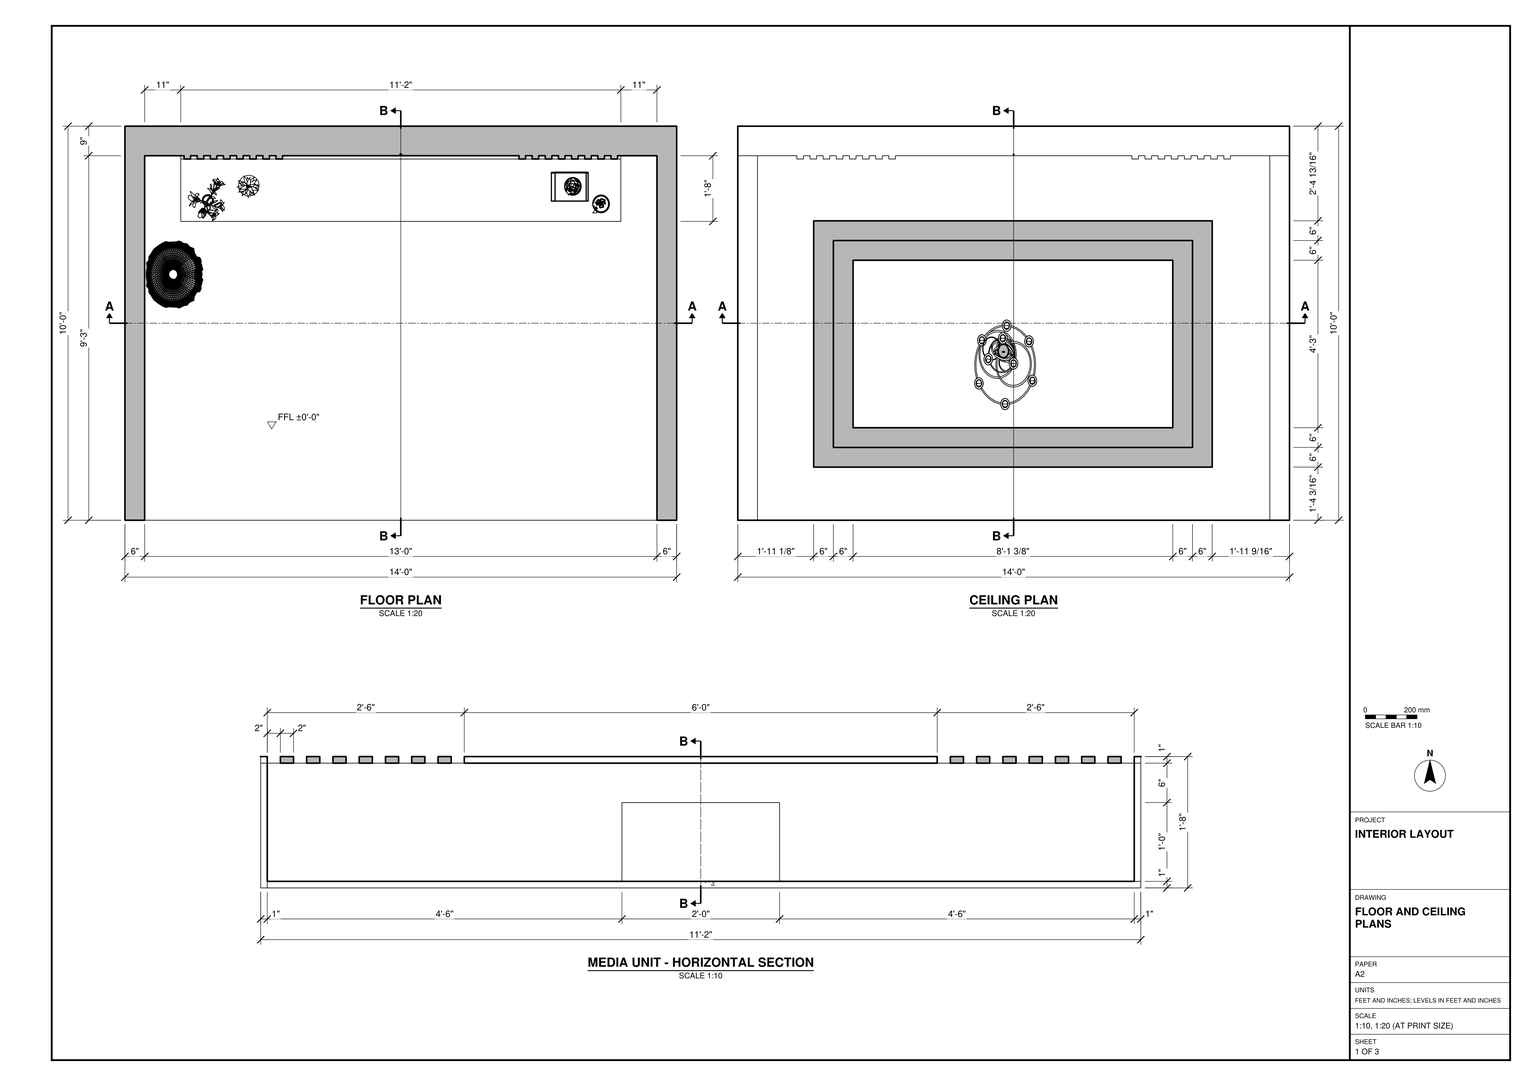
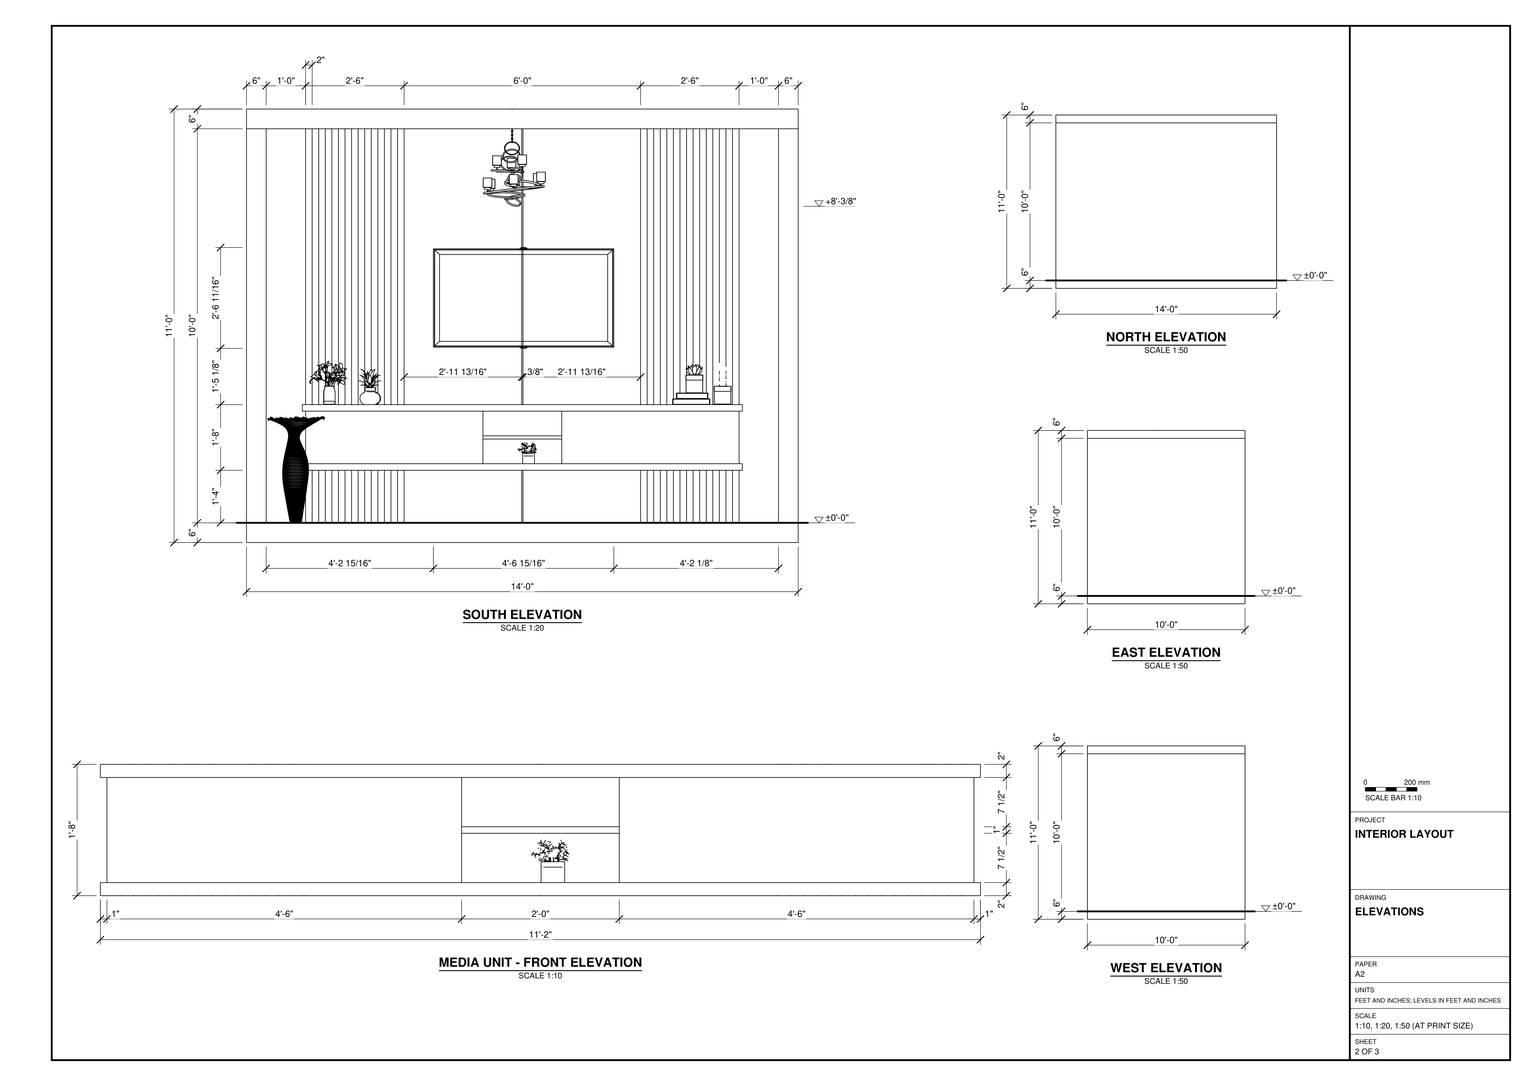
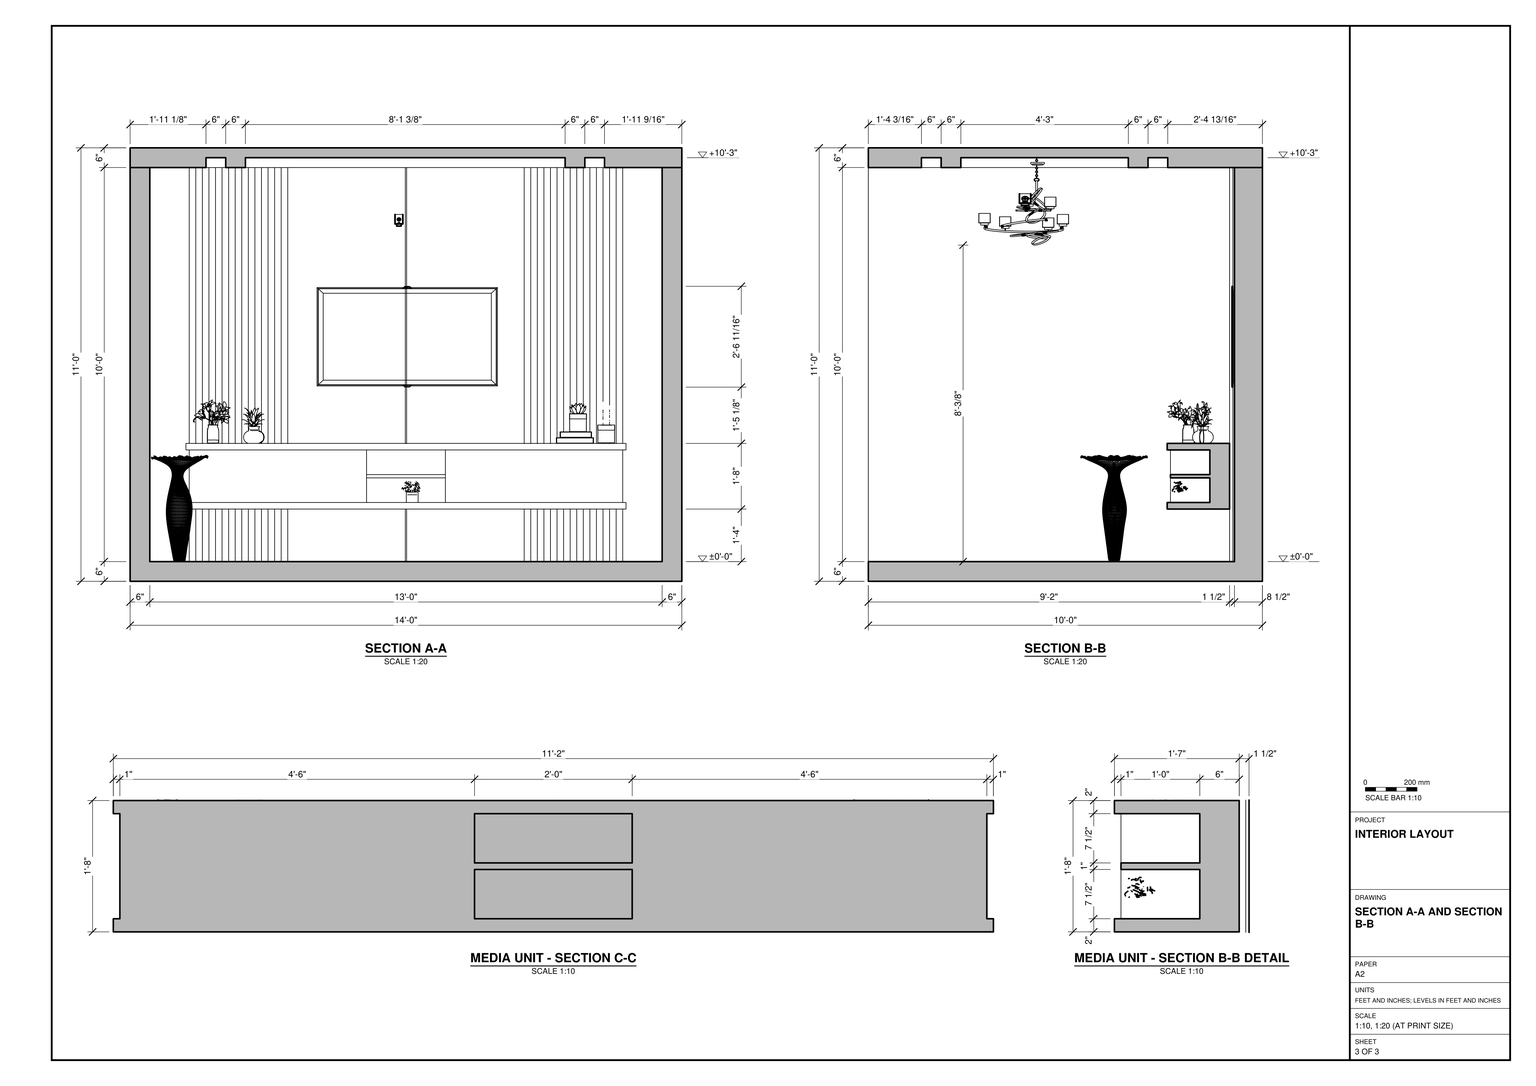
Build the room in SketchUp from task_files/diagram_01.pdf. Work in feet and inches. The room is 14'-0" wide, 10'-0" deep and 11'-0" high overall. Use the finished floor at ±0'-0" as the datum. Model the floor slab, the two 6" side walls and the rear wall assembly shown as 9" thick in plan. Leave the front open as drawn. Shape the underside of the ceiling slab to form the rectangular recess and its stepped border, following the ceiling plan and both sections.

On the rear wall, place the screen on the broad central panel between fields of vertical slats. Continue the panel and slat pattern below the floating media unit. Centre the 11'-2" unit across the wall with its underside 1'-4" above the finished floor. Use the enlarged joinery details to set out the projecting top and bottom boards, the broad side bays and the shelf dividing the open middle bay. Place the hanging light in the ceiling recess, the floor vase to the left of the unit and the smaller display items as shown in elevation. Decor and loose items may be any suitable library components.

Keep the walls, floor slab and ceiling slab as separate groups or components, and do the same for each furniture or joinery piece. Use components for repeated parts such as the slats. Save one SketchUp model as output_files/media_room_with_floating_joinery_and_a_recessed_ceiling.skp.

# SketchUp Ruby script. Lengths in inches.
U = 1.inch
M = Sketchup.active_model
def pt(a) = Geom::Point3d.new(a.map { |v| v * U })
def face(e, loops, mat)
  f = e.add_face(loops[0].map { |a| pt(a) })
  loops[1..].each { |l| e.add_face(l.map { |a| pt(a) }).erase! }
  f.material = f.back_material = mat if mat
  f
end
# faces: each face lists its corners as indices into pts; further lists are holes
def faces(e, pts, list, mat = nil) = list.each { |f| face(e, (f[0].is_a?(Array) ? f : [f]).map { |l| l.map { |i| pts[i] } }, mat) }
# xy, xz, yz: faces in a plane at the given z, y or x. An outline is a flat list of corners, or four numbers for a rectangle; further outlines are holes
def ring(l) = l.size == 4 ? [[l[0], l[1]], [l[2], l[1]], [l[2], l[3]], [l[0], l[3]]] : l.each_slice(2).to_a
def flat(e, list, mat, &to3) = list.each { |f| face(e, (f[0].is_a?(Array) ? f : [f]).map { |l| ring(l).map { |u, v| to3.(u, v) } }, mat) }
def xy(e, z, list, mat = nil) = flat(e, list, mat) { |x, y| [x, y, z] }
def xz(e, y, list, mat = nil) = flat(e, list, mat) { |x, z| [x, y, z] }
def yz(e, x, list, mat = nil) = flat(e, list, mat) { |y, z| [x, y, z] }
def lines(e, pts, list) = list.each { |a, b| e.add_line(pt(pts[a]), pt(pts[b])) }
# prism: a flat outline (further loops are holes) pulled along v
def prism(e, loops, v, mat = nil)
  f = face(e, loops, mat); d = Geom::Vector3d.new(v.map { |x| x * U })
  f.pushpull(f.normal.samedirection?(d) ? d.length : -d.length)
end
def box(e, o, s, mat = nil) = prism(e, [[o, [o[0] + s[0], o[1], o[2]], [o[0] + s[0], o[1] + s[1], o[2]], [o[0], o[1] + s[1], o[2]]]], [0, 0, s[2]], mat)
def at(x, y, z, deg = 0) = Geom::Transformation.translation(pt([x, y, z])) * Geom::Transformation.rotation(ORIGIN, Z_AXIS, deg.degrees)
def axes(o, x, y, z) = Geom::Transformation.new([*x, 0, *y, 0, *z, 0, *pt(o).to_a, 1])
def part(name) = M.definitions.add(name)
# library, detail: a bought-in or finely detailed component or shape, given as its bounding box
def library(name, o, s) = part(name).tap { |d| box(d.entities, o, s) }
def detail(e, o, s) = box(e.add_group.entities, o, s)
def put(e, d, t, mat = nil) = e.add_instance(d, t).tap { |i| i.material = mat if mat }
def group(e, t, mat = nil) = e.add_group.tap { |g| g.transformation = t; g.material = mat if mat }.entities
root = M.entities
M.materials.add("[0030_OldLace]").color = [253, 245, 230]
M.materials.add("[Carrera Marble]").color = [207, 207, 207]
M.materials.add("[Wood Bamboo]").color = [177, 105, 43]
c1 = library("Flat screen television",[0,1.41,1.14],[35.92,0.28,20.21])
c2 = library("Mint+Plant",[-0.84,-3.51,-0.07],[7.9,7.03,9.76])
c3 = library("suculentas com livro",[0,-0.27,0],[14.84,10.07,7.14])
c4 = library("lọ hoa",[2.76,5.43,0],[11.3,13.25,13.27])
c5 = library("MORNING+GLORY_AQUA",[22.86,12.49,0.11],[41.56,45.92,85.24])
c6 = library("Group_432",[-8.27,-1.37,0],[9.69,9.67,11.03])
c7 = library("Dalen+Chandelier",[-1.89,-23.41,-0.83],[35.87,36,58.86])
xy(root,126,[[[0,0,168,120],[23.11,16.17,144.46,91.17]],[[29.11,22.17,138.46,85.17],[35.11,28.17,132.46,79.17]]],"[0030_OldLace]")
xy(root,129,[[[23.11,16.17,144.46,91.17],[29.11,22.17,138.46,85.17]],[35.11,28.17,132.46,79.17]],"[0030_OldLace]")
xy(root,132,[[0,0,168,120]],"[0030_OldLace]")
xz(root,0,[[0,126,168,132]],"[0030_OldLace]")
xz(root,16.17,[[23.11,126,144.46,129]],"[0030_OldLace]")
xz(root,22.17,[[29.11,126,138.46,129]],"[0030_OldLace]")
xz(root,28.17,[[35.11,126,132.46,129]],"[0030_OldLace]")
xz(root,79.17,[[35.11,126,132.46,129]],"[0030_OldLace]")
xz(root,85.17,[[29.11,126,138.46,129]],"[0030_OldLace]")
xz(root,91.17,[[23.11,126,144.46,129]],"[0030_OldLace]")
xz(root,120,[[0,126,168,132]],"[0030_OldLace]")
yz(root,0,[[0,126,120,132]],"[0030_OldLace]")
yz(root,23.11,[[16.17,126,91.17,129]],"[0030_OldLace]")
yz(root,29.11,[[22.17,126,85.17,129]],"[0030_OldLace]")
yz(root,35.11,[[28.17,126,79.17,129]],"[0030_OldLace]")
yz(root,132.46,[[28.17,126,79.17,129]],"[0030_OldLace]")
yz(root,138.46,[[22.17,126,85.17,129]],"[0030_OldLace]")
yz(root,144.46,[[16.17,126,91.17,129]],"[0030_OldLace]")
yz(root,168,[[0,126,120,132]],"[0030_OldLace]")
put(root,c1,axes([56.91,109.3125,57.4],[1.52975,0,0],[0,1,0],[0,0,1.5196]))
put(root,c2,axes([83.13,94.06,24.05],[0.78,0,0],[0,0.87,0],[0,0,0.69]))
put(root,c3,axes([129.76,93.57,42],[1.2,0,0],[0,1.27693,0],[0,0,2]))
put(root,c4,at(16.47,85.57,42))
put(root,c5,axes([-3.04,59.05,5.96],[0.416,0,0],[0,0.445,0],[0,0,0.38]))
put(root,c6,at(40.92,98.19,42))
put(root,c7,axes([71.87,51.53,102.26],[0.59559,0,0],[0,0.77552,0],[0,0,0.51254]))
g1 = group(root,at(0,0,0),"[0030_OldLace]")
xy(g1,0,[[0,0,168,120]])
xy(g1,6,[[6,0,162,0,162,111,150,111,150,110,148,110,148,111,146,111,146,110,144,110,144,111,142,111,142,110,140,110,140,111,138,111,138,110,136,110,136,111,134,111,134,110,132,110,132,111,130,111,130,110,128,110,128,111,126,111,126,110,124,110,124,111,122,111,122,110,120,110,120,111,84.2,111,84.2,111.5,83.8,111.5,83.8,111,48,111,48,110,46,110,46,111,44,111,44,110,42,110,42,111,40,111,40,110,38,110,38,111,36,111,36,110,34,110,34,111,32,111,32,110,30,110,30,111,28,111,28,110,26,110,26,111,24,111,24,110,22,110,22,111,20,111,20,110,18,110,18,111,6,111]],"[Carrera Marble]")
xy(g1,22,[[17,110,18,111],[150,110,151,111]])
xy(g1,22,[[17,91,151,110]],"[Wood Bamboo]")
xy(g1,24,[[17,91,18,110],[18,91,151,91,151,92,96,92,96,104,72,104,72,92,18,92],[150,92,151,110],[17,110,18,111],[150,110,151,111]],"[Wood Bamboo]")
xy(g1,31.5,[[72,92,96,104]],"[Wood Bamboo]")
xy(g1,32.5,[[72,92,96,104]],"[Wood Bamboo]")
xy(g1,40,[[17,92,18,110],[17,110,18,111]])
xy(g1,40,[[17,91,17,92,72,92,72,104,96,104,96,92,151,92,151,91],[150,92,151,110],[150,110,151,111]],"[Wood Bamboo]")
xy(g1,42,[[150,110,151,111]])
xy(g1,42,[[17,91,151,110],[17,110,18,111]],"[Wood Bamboo]")
xy(g1,126,[[18,110,20,110,20,111,22,111,22,110,24,110,24,111,26,111,26,110,28,110,28,111,30,111,30,110,32,110,32,111,34,111,34,110,36,110,36,111,38,111,38,110,40,110,40,111,42,111,42,110,44,110,44,111,46,111,46,110,48,110,48,111,83.8,111,83.8,111.5,84.2,111.5,84.2,111,120,111,120,110,122,110,122,111,124,111,124,110,126,110,126,111,128,111,128,110,130,110,130,111,132,111,132,110,134,110,134,111,136,111,136,110,138,110,138,111,140,111,140,110,142,110,142,111,144,111,144,110,146,110,146,111,148,111,148,110,150,110,150,111,168,111,168,120,0,120,0,111,18,111]])
xy(g1,126,[[0,0,6,111],[162,0,168,111]],"[Carrera Marble]")
xz(g1,0,[[0,0,168,0,168,126,162,126,162,6,6,6,6,126,0,126]])
xz(g1,91,[[17,22,151,24],[17,40,151,42]],"[Wood Bamboo]")
xz(g1,92,[[18,24,72,40],[96,24,150,40]],"[0030_OldLace]")
xz(g1,92,[[72,31.5,96,32.5]],"[Wood Bamboo]")
xz(g1,104,[[72,24,96,31.5],[72,32.5,96,40]],"[0030_OldLace]")
xz(g1,110,[[20,22,22,42],[24,22,26,42],[28,22,30,42],[32,22,34,42],[36,22,38,42],
  [40,22,42,42],[44,22,46,42],[48,22,120,42],[122,22,124,42],[126,22,128,42],
  [130,22,132,42],[134,22,136,42],[138,22,140,42],[142,22,144,42],[146,22,148,42]])
xz(g1,110,[[18,6,20,22],[22,6,24,22],[26,6,28,22],[30,6,32,22],[34,6,36,22],
  [38,6,40,22],[42,6,44,22],[46,6,48,22],[120,6,122,22],[124,6,126,22],
  [128,6,130,22],[132,6,134,22],[136,6,138,22],[140,6,142,22],[144,6,146,22],
  [148,6,150,22],[18,42,20,126],[22,42,24,126],[26,42,28,126],[30,42,32,126],
  [34,42,36,126],[38,42,40,126],[42,42,44,126],[46,42,48,126],[120,42,122,126],
  [124,42,126,126],[128,42,130,126],[132,42,134,126],[136,42,138,126],[140,42,142,126],
  [144,42,146,126],[148,42,150,126]],"[Wood Bamboo]")
xz(g1,111,[[48,6,83.8,126],[84.2,6,120,126]],"[0030_OldLace]")
xz(g1,111,[[6,6,18,6,18,22,17,22,17,24,18,24,18,40,17,40,17,42,18,42,18,126,6,126],[150,6,162,6,162,126,150,126,150,42,151,42,151,40,150,40,150,24,151,24,151,22,150,22]],"[Carrera Marble]")
xz(g1,111,[[20,6,22,126],[24,6,26,126],[28,6,30,126],[32,6,34,126],[36,6,38,126],
  [40,6,42,126],[44,6,46,126],[122,6,124,126],[126,6,128,126],[130,6,132,126],
  [134,6,136,126],[138,6,140,126],[142,6,144,126],[146,6,148,126]],"[Wood Bamboo]")
xz(g1,111.5,[[83.8,6,84.2,126]],"[0030_OldLace]")
xz(g1,120,[[0,0,168,126]])
yz(g1,0,[[0,0,120,126]])
yz(g1,6,[[0,6,111,126]],"[Carrera Marble]")
yz(g1,17,[[91,22,111,24],[91,40,111,42]],"[Wood Bamboo]")
yz(g1,18,[[92,24,111,40]],"[0030_OldLace]")
yz(g1,18,[[110,6,111,22],[110,42,111,126]],"[Wood Bamboo]")
yz(g1,20,[[110,6,111,126]],"[Wood Bamboo]")
yz(g1,22,[[110,6,111,126]],"[Wood Bamboo]")
yz(g1,24,[[110,6,111,126]],"[Wood Bamboo]")
yz(g1,26,[[110,6,111,126]],"[Wood Bamboo]")
yz(g1,28,[[110,6,111,126]],"[Wood Bamboo]")
yz(g1,30,[[110,6,111,126]],"[Wood Bamboo]")
yz(g1,32,[[110,6,111,126]],"[Wood Bamboo]")
yz(g1,34,[[110,6,111,126]],"[Wood Bamboo]")
yz(g1,36,[[110,6,111,126]],"[Wood Bamboo]")
yz(g1,38,[[110,6,111,126]],"[Wood Bamboo]")
yz(g1,40,[[110,6,111,126]],"[Wood Bamboo]")
yz(g1,42,[[110,6,111,126]],"[Wood Bamboo]")
yz(g1,44,[[110,6,111,126]],"[Wood Bamboo]")
yz(g1,46,[[110,6,111,126]],"[Wood Bamboo]")
yz(g1,48,[[110,6,111,126]],"[Wood Bamboo]")
yz(g1,72,[[92,24,104,31.5],[92,32.5,104,40]],"[0030_OldLace]")
yz(g1,83.8,[[111,6,111.5,126]],"[0030_OldLace]")
yz(g1,84.2,[[111,6,111.5,126]],"[0030_OldLace]")
yz(g1,96,[[92,24,104,31.5],[92,32.5,104,40]],"[0030_OldLace]")
yz(g1,120,[[110,6,111,126]],"[Wood Bamboo]")
yz(g1,122,[[110,6,111,126]],"[Wood Bamboo]")
yz(g1,124,[[110,6,111,126]],"[Wood Bamboo]")
yz(g1,126,[[110,6,111,126]],"[Wood Bamboo]")
yz(g1,128,[[110,6,111,126]],"[Wood Bamboo]")
yz(g1,130,[[110,6,111,126]],"[Wood Bamboo]")
yz(g1,132,[[110,6,111,126]],"[Wood Bamboo]")
yz(g1,134,[[110,6,111,126]],"[Wood Bamboo]")
yz(g1,136,[[110,6,111,126]],"[Wood Bamboo]")
yz(g1,138,[[110,6,111,126]],"[Wood Bamboo]")
yz(g1,140,[[110,6,111,126]],"[Wood Bamboo]")
yz(g1,142,[[110,6,111,126]],"[Wood Bamboo]")
yz(g1,144,[[110,6,111,126]],"[Wood Bamboo]")
yz(g1,146,[[110,6,111,126]],"[Wood Bamboo]")
yz(g1,148,[[110,6,111,126]],"[Wood Bamboo]")
yz(g1,150,[[92,24,111,40]],"[0030_OldLace]")
yz(g1,150,[[110,6,111,22],[110,42,111,126]],"[Wood Bamboo]")
yz(g1,151,[[91,22,111,24],[91,40,111,42]],"[Wood Bamboo]")
yz(g1,162,[[0,6,111,126]],"[Carrera Marble]")
yz(g1,168,[[0,0,120,126]])
p = [[164.79,117.13,0],[162,111,6]]
lines(g1,p,[[0,1]])
